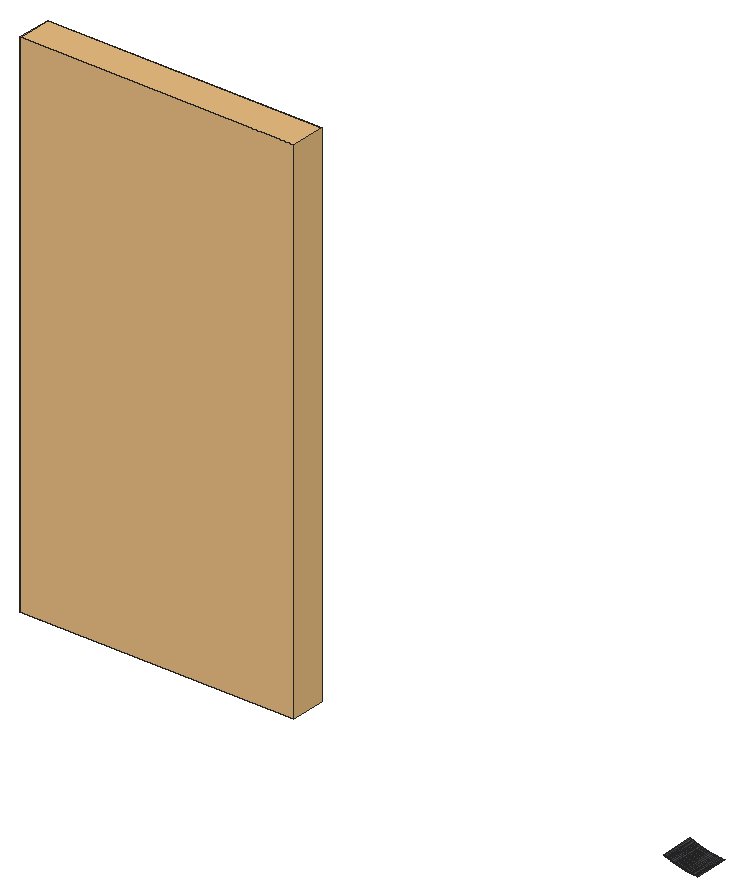
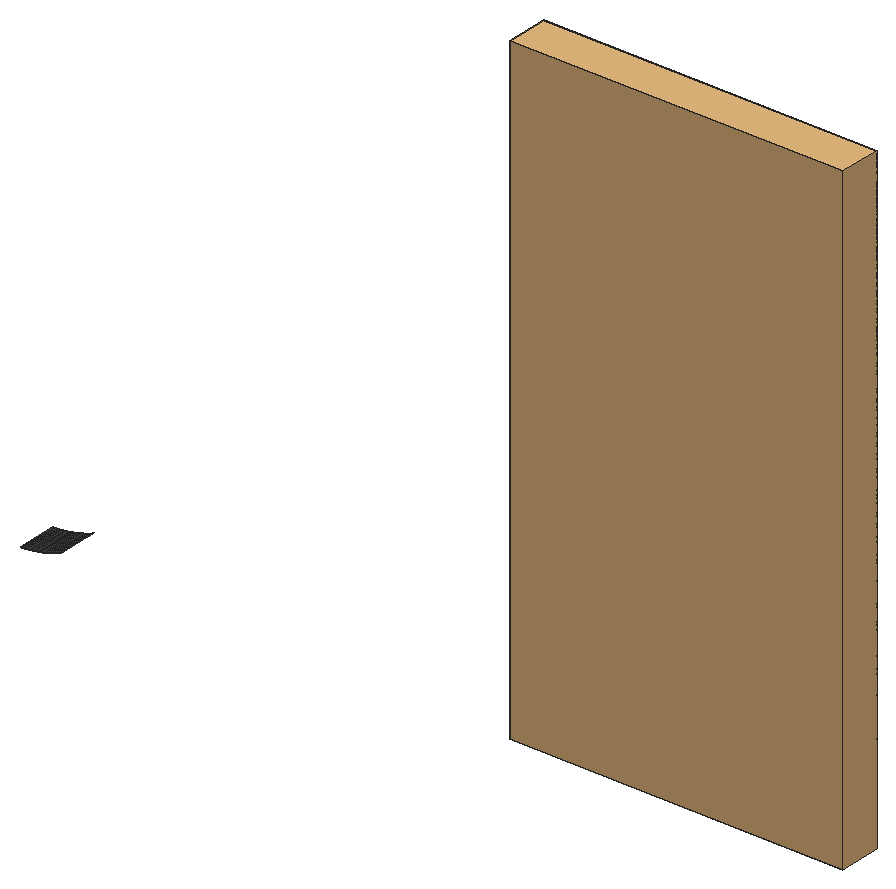
# SketchUp Ruby script. Lengths in inches.
U = 1.inch
M = Sketchup.active_model
def pt(a) = Geom::Point3d.new(a.map { |v| v * U })
def face(e, loops, mat)
  f = e.add_face(loops[0].map { |a| pt(a) })
  loops[1..].each { |l| e.add_face(l.map { |a| pt(a) }).erase! }
  f.material = f.back_material = mat if mat
  f
end
# faces: each face lists its corners as indices into pts; further lists are holes
def faces(e, pts, list, mat = nil) = list.each { |f| face(e, (f[0].is_a?(Array) ? f : [f]).map { |l| l.map { |i| pts[i] } }, mat) }
# xy, xz, yz: faces in a plane at the given z, y or x. An outline is a flat list of corners, or four numbers for a rectangle; further outlines are holes
def ring(l) = l.size == 4 ? [[l[0], l[1]], [l[2], l[1]], [l[2], l[3]], [l[0], l[3]]] : l.each_slice(2).to_a
def flat(e, list, mat, &to3) = list.each { |f| face(e, (f[0].is_a?(Array) ? f : [f]).map { |l| ring(l).map { |u, v| to3.(u, v) } }, mat) }
def xy(e, z, list, mat = nil) = flat(e, list, mat) { |x, y| [x, y, z] }
def xz(e, y, list, mat = nil) = flat(e, list, mat) { |x, z| [x, y, z] }
def yz(e, x, list, mat = nil) = flat(e, list, mat) { |y, z| [x, y, z] }
def lines(e, pts, list) = list.each { |a, b| e.add_line(pt(pts[a]), pt(pts[b])) }
# prism: a flat outline (further loops are holes) pulled along v
def prism(e, loops, v, mat = nil)
  f = face(e, loops, mat); d = Geom::Vector3d.new(v.map { |x| x * U })
  f.pushpull(f.normal.samedirection?(d) ? d.length : -d.length)
end
def box(e, o, s, mat = nil) = prism(e, [[o, [o[0] + s[0], o[1], o[2]], [o[0] + s[0], o[1] + s[1], o[2]], [o[0], o[1] + s[1], o[2]]]], [0, 0, s[2]], mat)
def at(x, y, z, deg = 0) = Geom::Transformation.translation(pt([x, y, z])) * Geom::Transformation.rotation(ORIGIN, Z_AXIS, deg.degrees)
def axes(o, x, y, z) = Geom::Transformation.new([*x, 0, *y, 0, *z, 0, *pt(o).to_a, 1])
def part(name) = M.definitions.add(name)
# library, detail: a bought-in or finely detailed component or shape, given as its bounding box
def library(name, o, s) = part(name).tap { |d| box(d.entities, o, s) }
def detail(e, o, s) = box(e.add_group.entities, o, s)
def put(e, d, t, mat = nil) = e.add_instance(d, t).tap { |i| i.material = mat if mat }
def group(e, t, mat = nil) = e.add_group.tap { |g| g.transformation = t; g.material = mat if mat }.entities
root = M.entities
M.materials.add("1432 AP 8245 TAR ROAD").color = [71, 72, 75]
M.materials.add("[Wood Veneer 01]").color = [120, 70, 37]
c1 = library("Group\#10",[-12,-12.5,-12],[99,12.5,186])
p = [[276.74,107.37,155.86],[277.02,107.37,155.85],[277.02,95.37,155.85],[276.74,95.37,155.86],[277.3,107.37,155.83],[277.3,95.37,155.83],
  [277.59,107.37,155.82],[277.59,95.37,155.82],[275.61,107.37,155.95],[275.89,107.37,155.93],[275.89,95.37,155.93],[275.61,95.37,155.95],
  [276.18,107.37,155.9],[276.18,95.37,155.9],[276.46,107.37,155.88],[276.46,95.37,155.88],[274.49,107.37,156.08],[274.77,107.37,156.04],
  [274.77,95.37,156.04],[274.49,95.37,156.08],[275.05,107.37,156.01],[275.05,95.37,156.01],[275.33,107.37,155.98],[275.33,95.37,155.98],
  [273.93,107.37,156.15],[274.21,107.37,156.11],[274.21,95.37,156.11],[273.93,95.37,156.15],[273.09,107.37,156.28],[273.37,107.37,156.24],
  [273.37,95.37,156.24],[273.09,95.37,156.28],[273.65,107.37,156.19],[273.65,95.37,156.19],[272.53,107.37,156.38],[272.8125,107.37,156.33],
  [272.8125,95.37,156.33],[272.53,95.37,156.38],[271.98,107.37,156.48],[272.25,107.37,156.43],[272.25,95.37,156.43],[271.98,95.37,156.48],
  [271.42,107.37,156.6],[271.7,107.37,156.54],[271.7,95.37,156.54],[271.42,95.37,156.6],[271.15,107.37,156.66],[271.15,95.37,156.66],
  [270.6,107.37,156.79],[270.87,107.37,156.72],[270.87,95.37,156.72],[270.6,95.37,156.79],[270.32,107.37,156.85],[270.32,95.37,156.85],
  [269.77,107.37,156.99],[270.05,107.37,156.92],[270.05,95.37,156.92],[269.77,95.37,156.99],[269.5,107.37,157.07],[269.5,95.37,157.07],
  [268.96,107.37,157.22],[269.23,107.37,157.14],[269.23,95.37,157.14],[268.96,95.37,157.22],[268.69,107.37,157.3],[268.69,95.37,157.3],
  [268.41,107.37,157.38],[268.41,95.37,157.38],[268.14,107.37,157.47],[268.14,95.37,157.47],[267.875,107.37,157.55],[267.875,95.37,157.55],
  [267.34,107.37,157.73],[267.61,107.37,157.64],[267.61,95.37,157.64],[267.34,95.37,157.73],[267.07,107.37,157.83],[267.07,95.37,157.83],
  [266.81,107.37,157.92],[266.81,95.37,157.92],[266.54,107.37,158.02],[266.54,95.37,158.02],[266.27,107.37,158.12],[266.27,95.37,158.12],
  [266.01,107.37,158.22],[266.01,95.37,158.22],[265.75,107.37,158.32],[265.75,95.37,158.32],[265.49,107.37,158.43],[265.49,95.37,158.43],
  [265.22,107.37,158.53],[265.22,95.37,158.53]]
faces(root,p,[[0,1,2,3],[1,4,5,2],[4,6,7,5],[8,9,10,11],[9,12,13,10],[12,14,15,13],[14,0,3,15],[16,17,18,19],
  [17,20,21,18],[20,22,23,21],[22,8,11,23],[24,25,26,27],[25,16,19,26],[28,29,30,31],[29,32,33,30],[32,24,27,33],
  [34,35,36,37],[35,28,31,36],[38,39,40,41],[39,34,37,40],[42,43,44,45],[43,38,41,44],[46,42,45,47],[48,49,50,51],
  [49,46,47,50],[52,48,51,53],[54,55,56,57],[55,52,53,56],[58,54,57,59],[60,61,62,63],[61,58,59,62],[64,60,63,65],
  [66,64,65,67],[68,66,67,69],[70,68,69,71],[72,73,74,75],[73,70,71,74],[76,72,75,77],[78,76,77,79],[80,78,79,81],
  [82,80,81,83],[84,82,83,85],[86,84,85,87],[88,86,87,89],[90,88,89,91]],"1432 AP 8245 TAR ROAD")
put(root,c1,at(45,107.37,167.79),"[Wood Veneer 01]")
